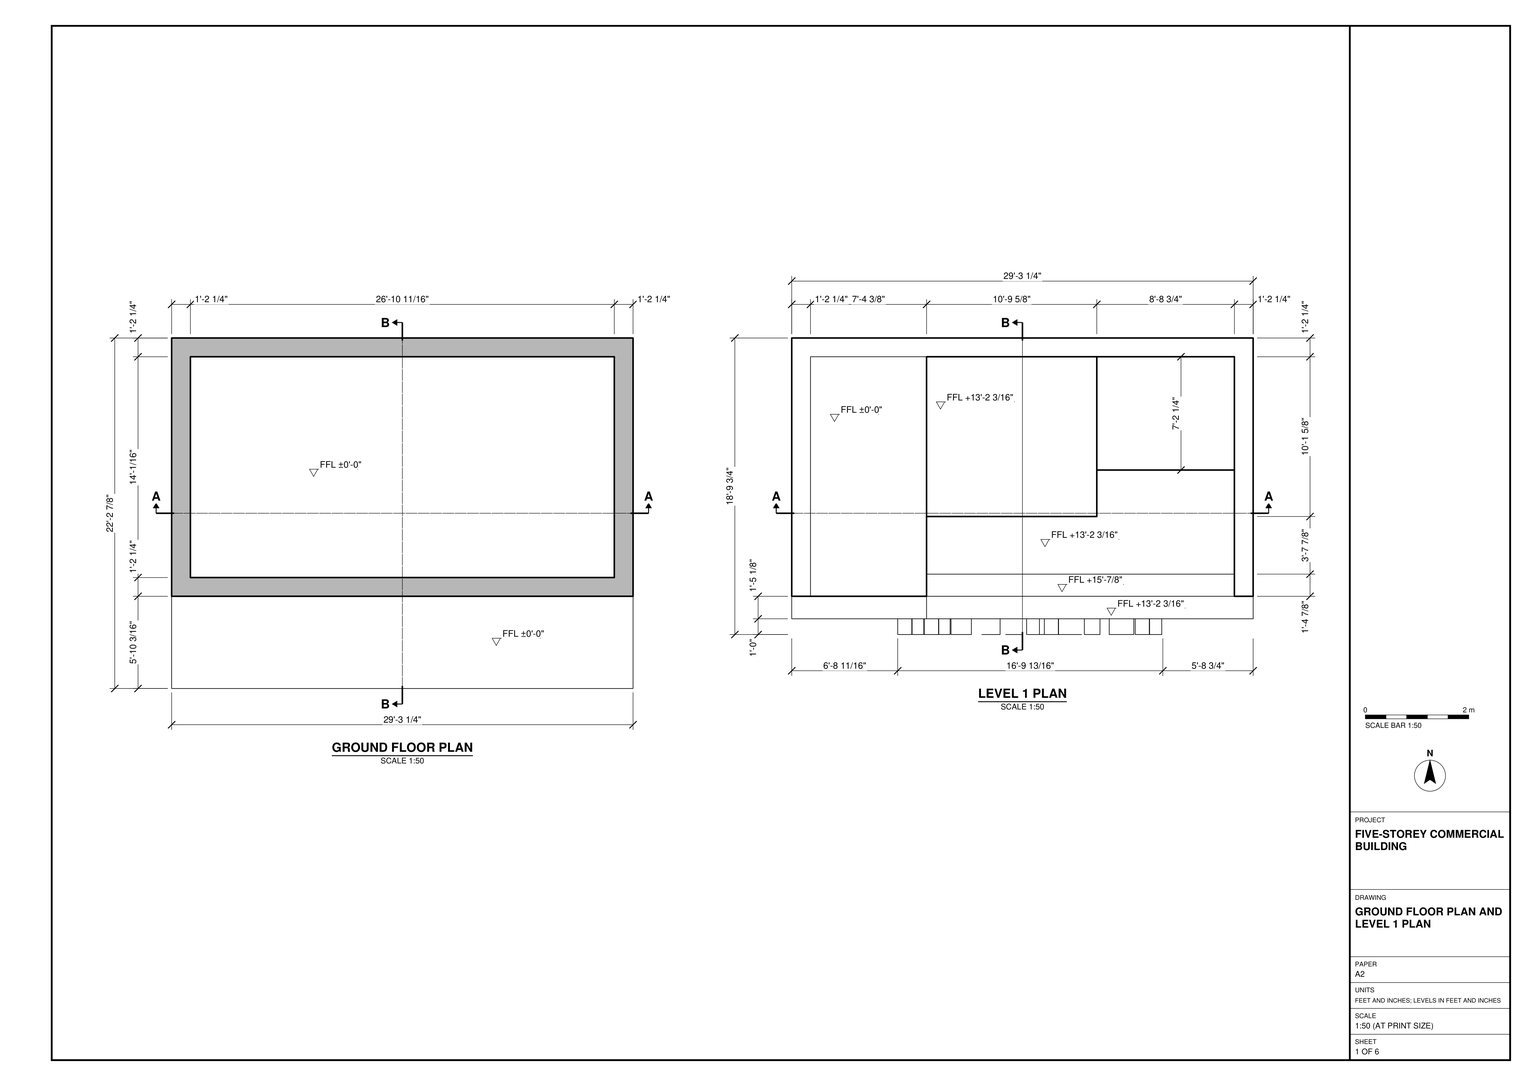
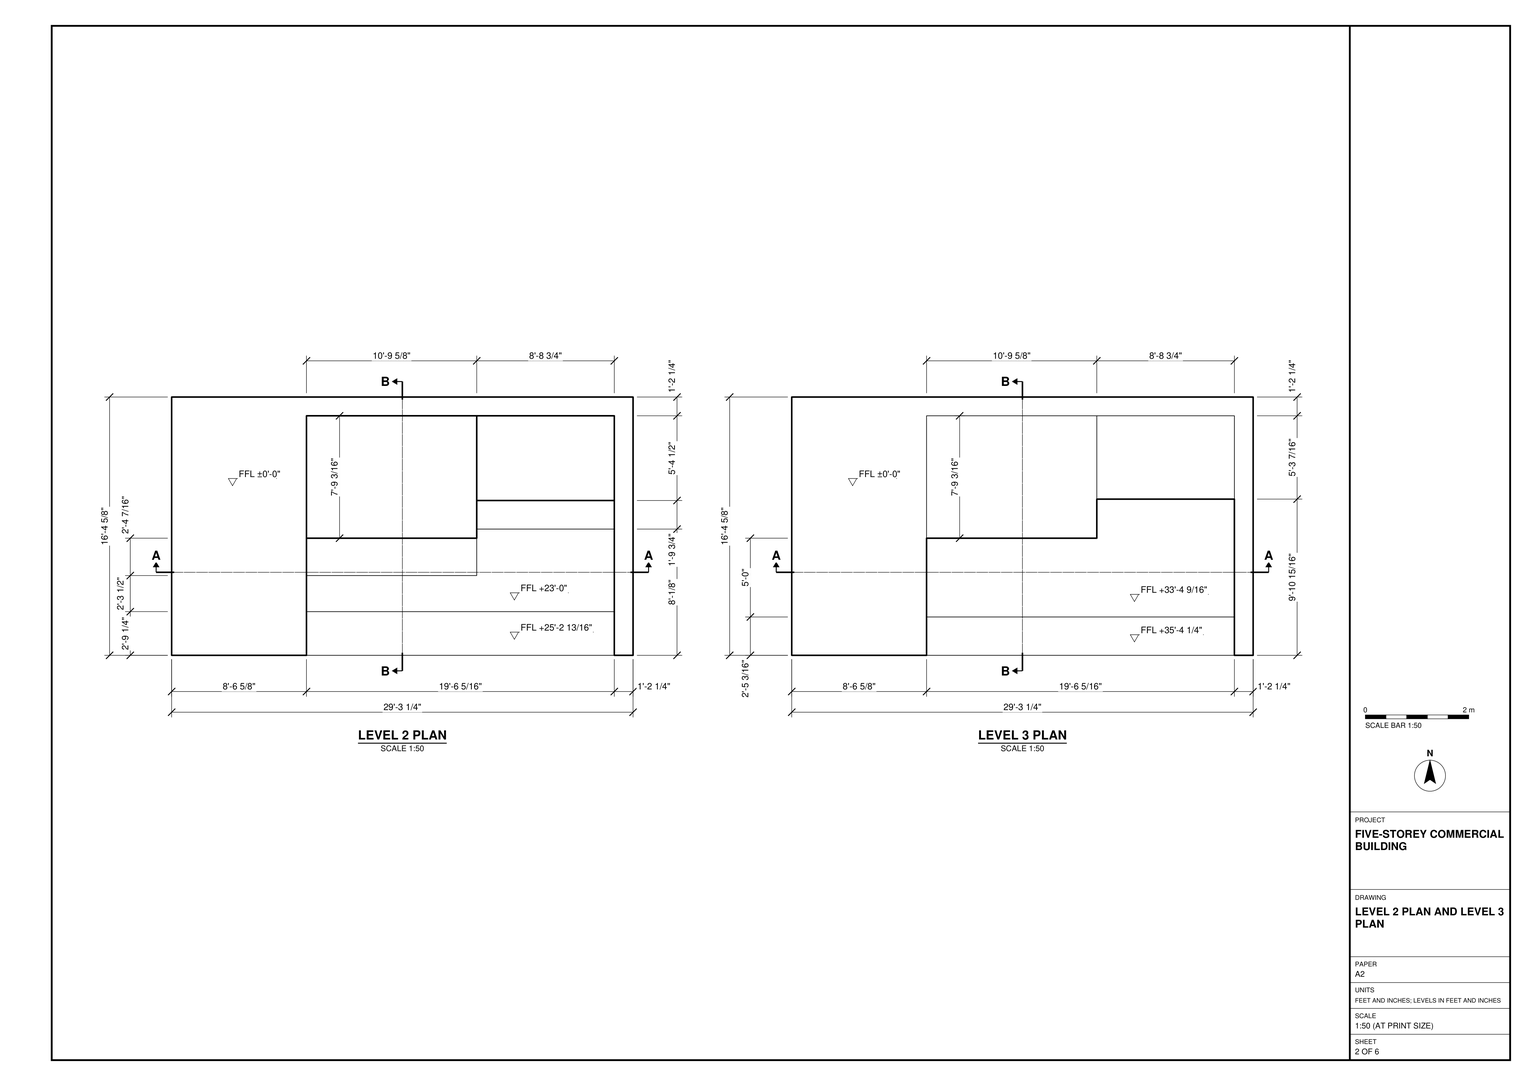
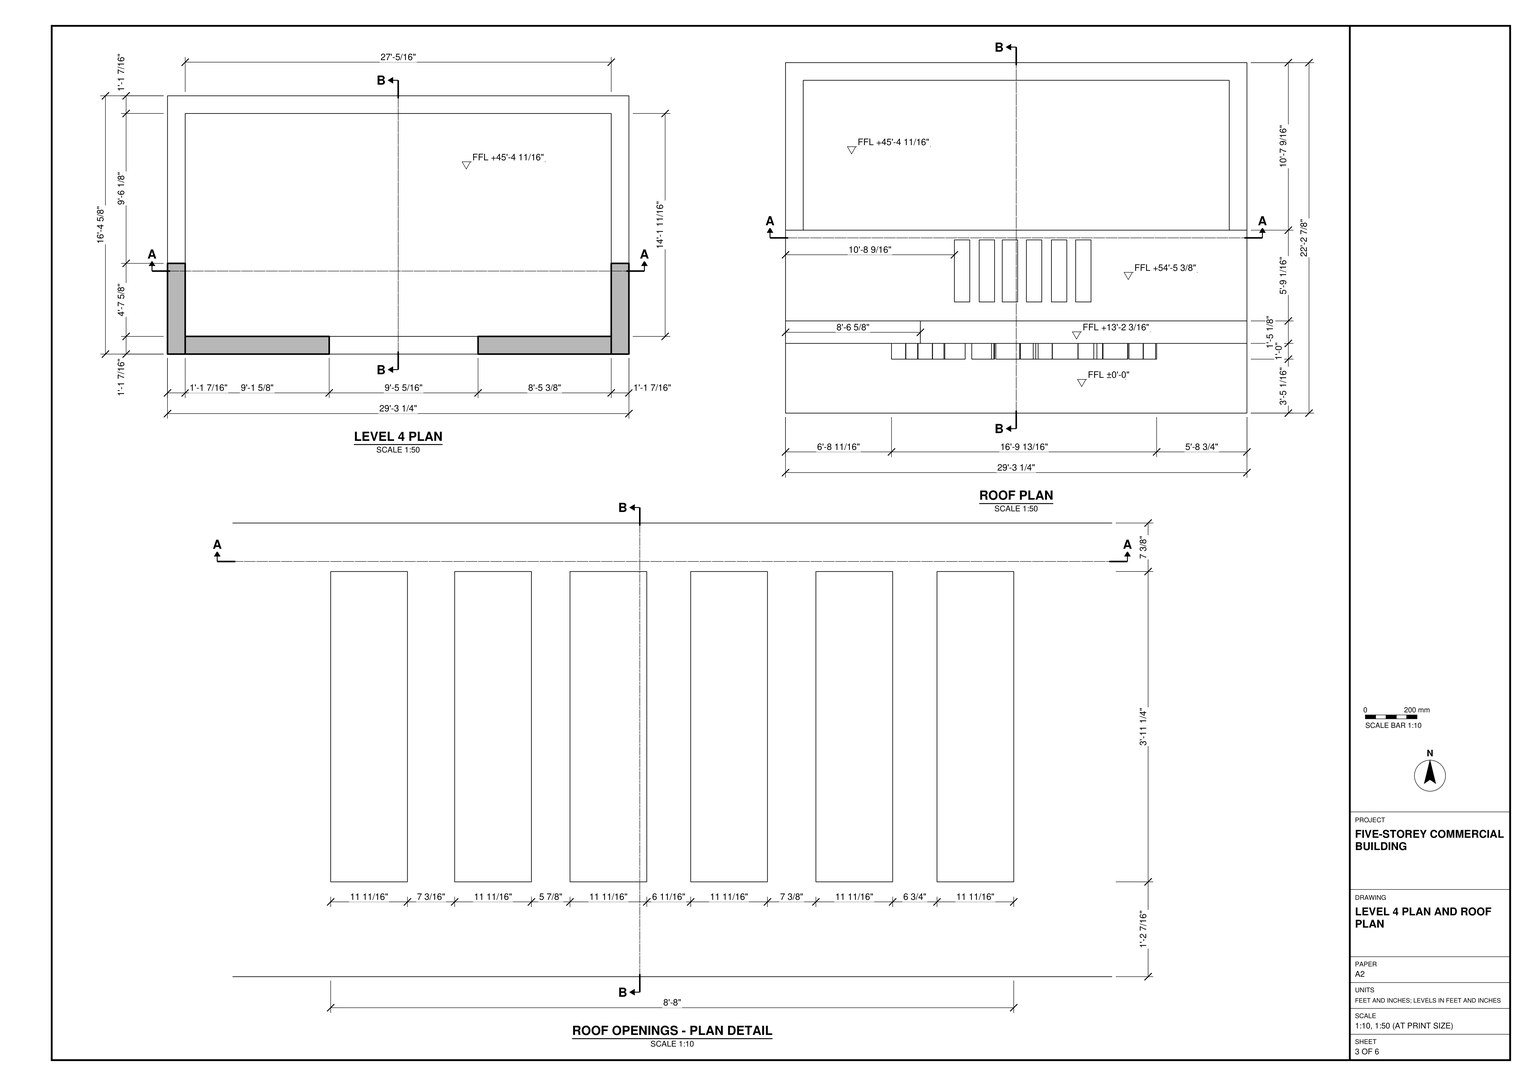
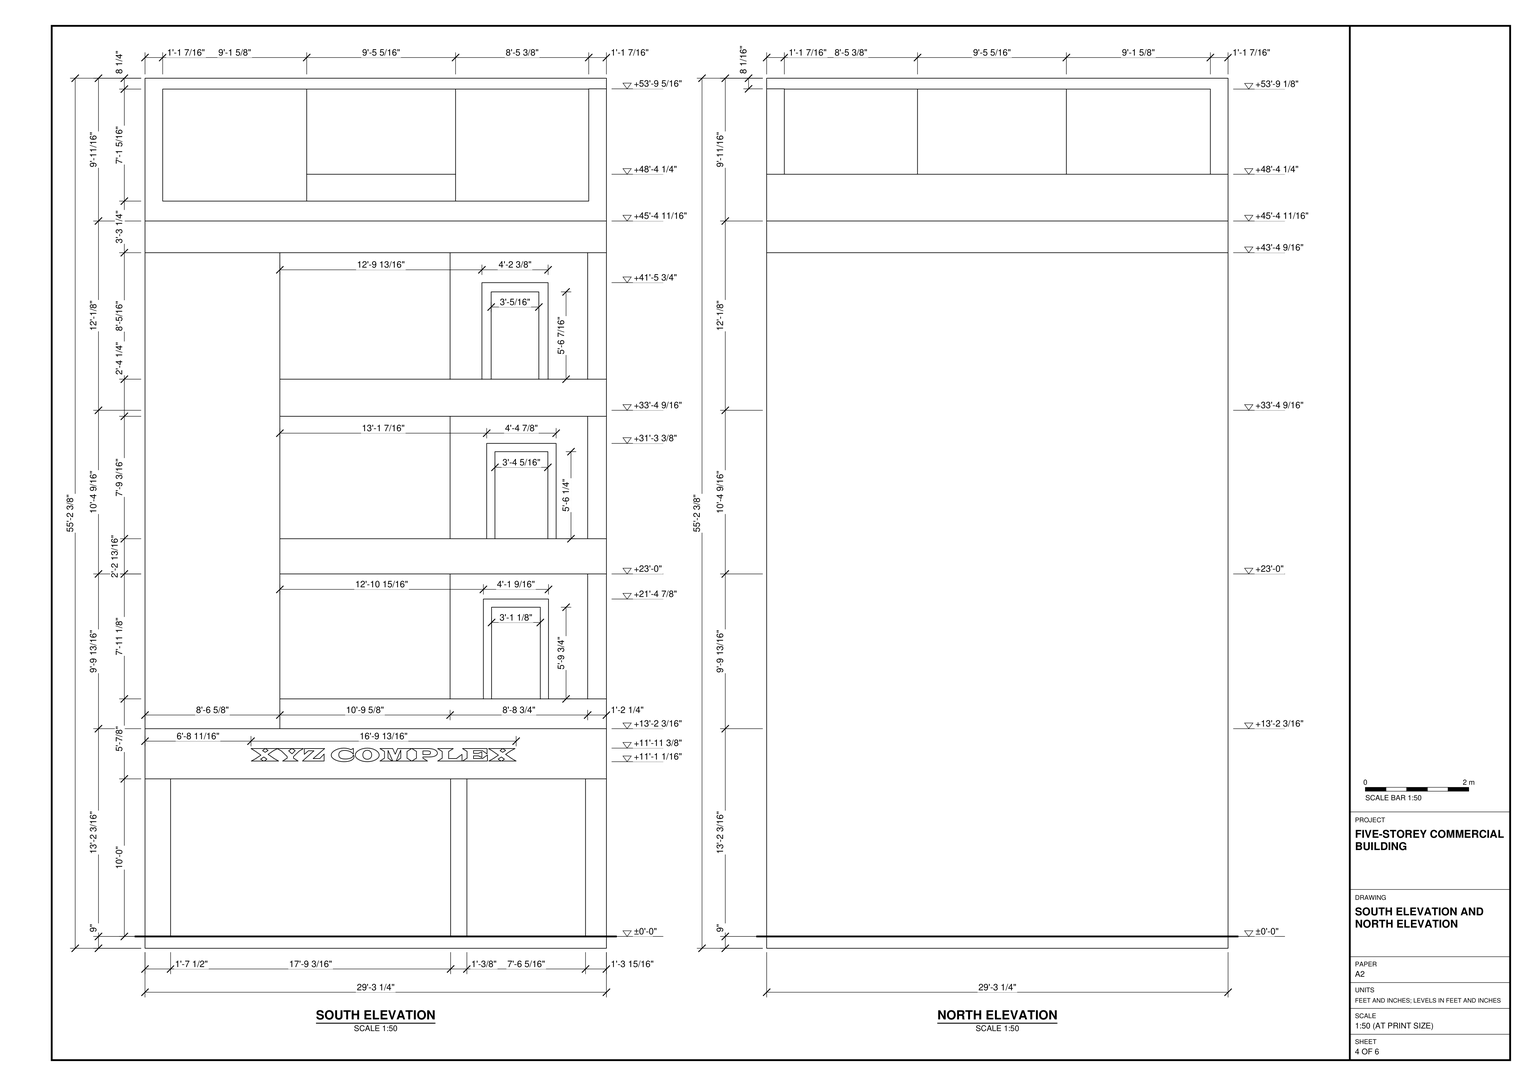
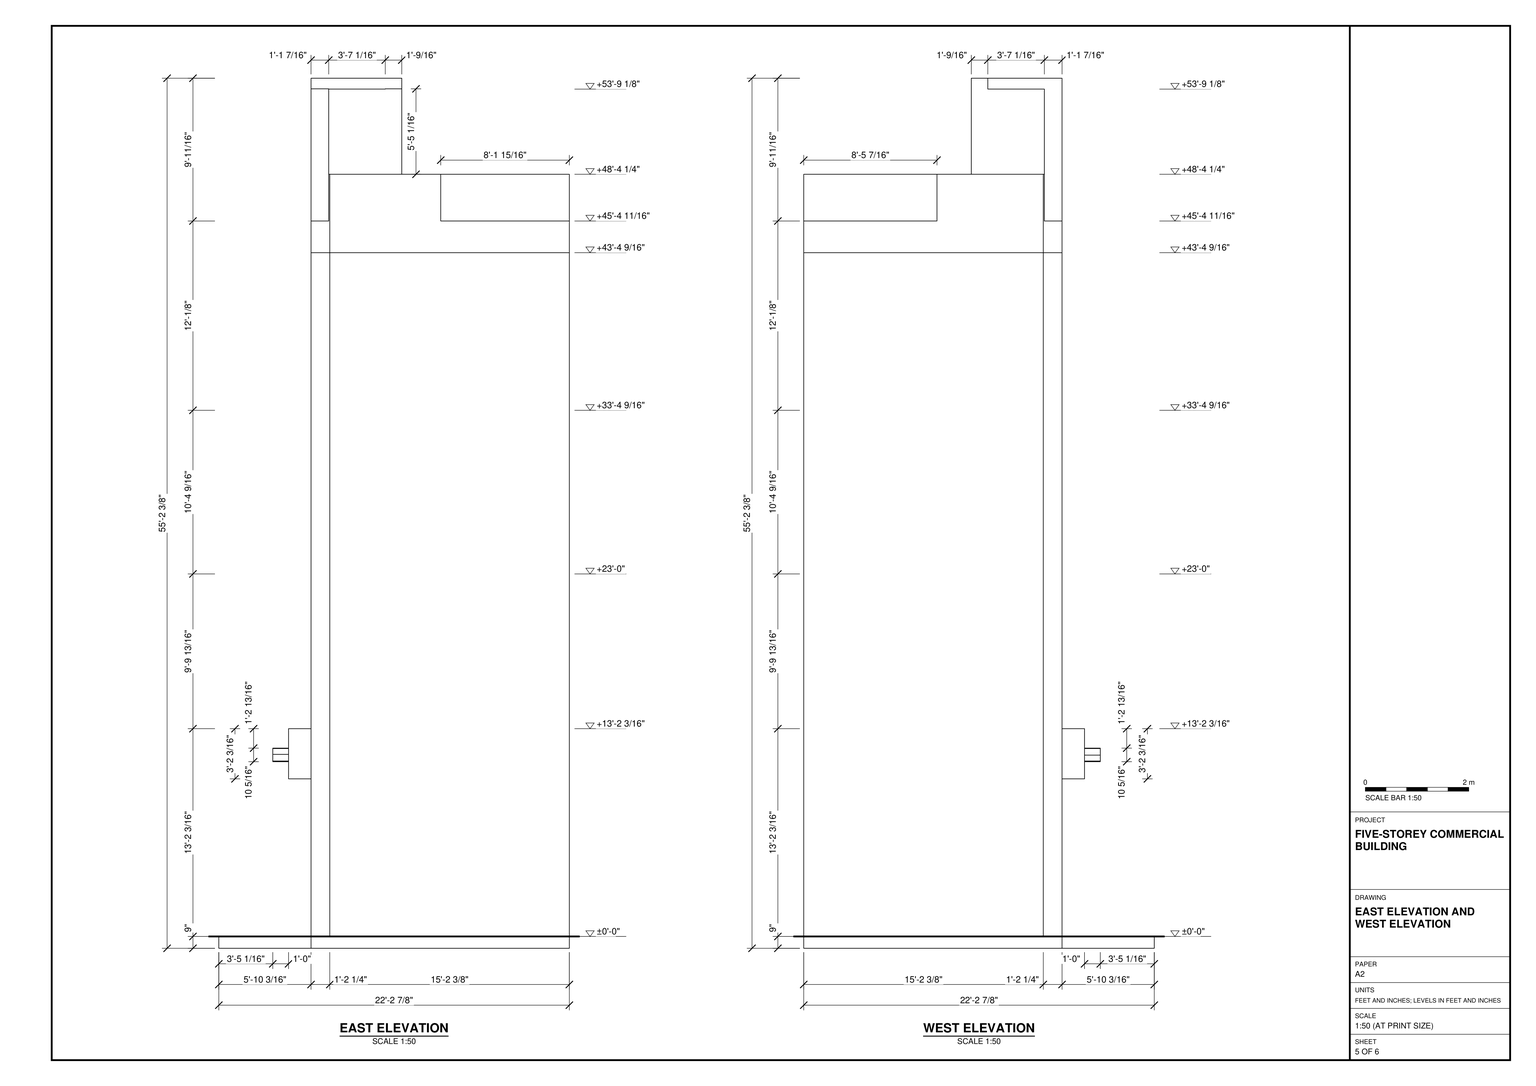
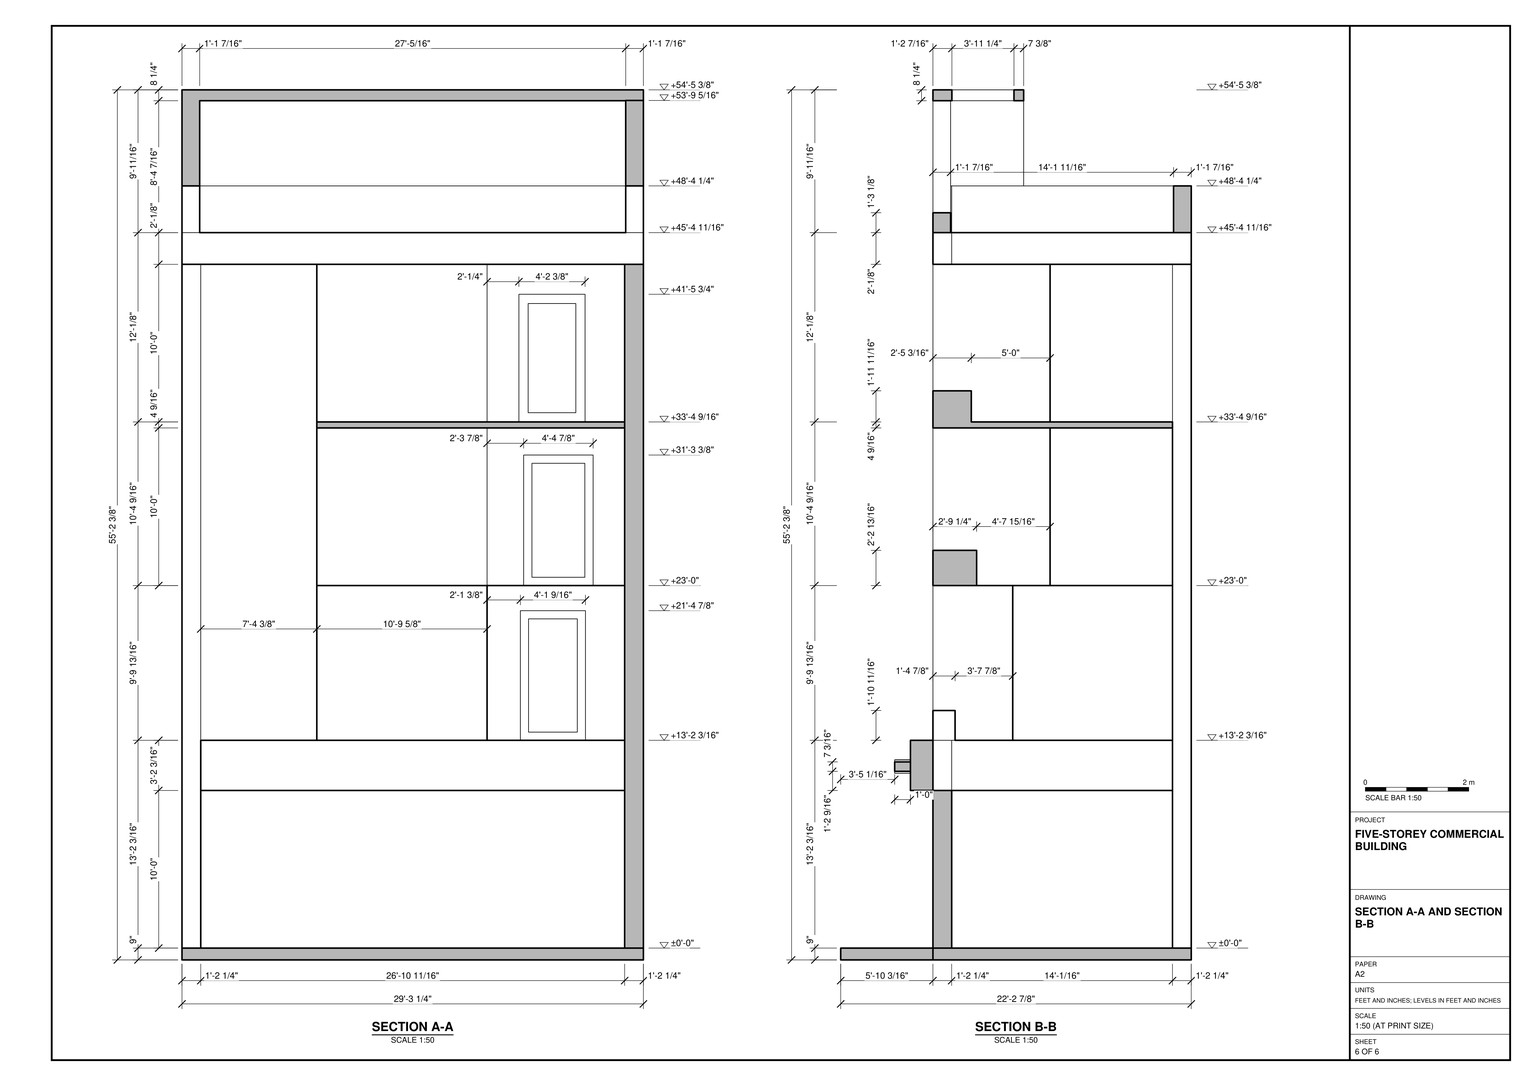
Use task_files/diagram_01.pdf to build the five-storey commercial building in SketchUp. Work in feet and inches. The overall width is 29'-3 1/4" along X, the depth is 22'-2 7/8" along Y, and the height is 55'-2 3/8" along Z. Set the ground floor at ±0'-0" and Levels 1 through 4 at +13'-2 3/16", +23'-0", +33'-4 9/16", and +45'-4 11/16", respectively.

Start with the rectangular ground-floor enclosure and extend the base in front of it as drawn. Use the wall thicknesses shown in plan. Model each slab from its own plan rather than copying a solid floor plate up the building. On Levels 1 through 3, keep the left-hand bay open to the ground floor and follow the changes in depth between the middle and right-hand bays. On Level 4, form the front corner walls and leave the gap between them. Use the enlarged roof detail to cut the six narrow rectangular openings in the front roof strip.

Follow the sheets for openings, stairs, built-in joinery and main furniture wherever shown. Keep walls, slabs, roof elements and each furniture or joinery piece in separate groups or components, and use components for repeated parts. Any decor or loose items shown may be suitable library components. Save one SketchUp model as output_files/five_storey_commercial_building_with_six_roof_openings.skp.

# SketchUp Ruby script. Lengths in inches.
U = 1.inch
M = Sketchup.active_model
def pt(a) = Geom::Point3d.new(a.map { |v| v * U })
def face(e, loops, mat)
  f = e.add_face(loops[0].map { |a| pt(a) })
  loops[1..].each { |l| e.add_face(l.map { |a| pt(a) }).erase! }
  f.material = f.back_material = mat if mat
  f
end
# faces: each face lists its corners as indices into pts; further lists are holes
def faces(e, pts, list, mat = nil) = list.each { |f| face(e, (f[0].is_a?(Array) ? f : [f]).map { |l| l.map { |i| pts[i] } }, mat) }
# xy, xz, yz: faces in a plane at the given z, y or x. An outline is a flat list of corners, or four numbers for a rectangle; further outlines are holes
def ring(l) = l.size == 4 ? [[l[0], l[1]], [l[2], l[1]], [l[2], l[3]], [l[0], l[3]]] : l.each_slice(2).to_a
def flat(e, list, mat, &to3) = list.each { |f| face(e, (f[0].is_a?(Array) ? f : [f]).map { |l| ring(l).map { |u, v| to3.(u, v) } }, mat) }
def xy(e, z, list, mat = nil) = flat(e, list, mat) { |x, y| [x, y, z] }
def xz(e, y, list, mat = nil) = flat(e, list, mat) { |x, z| [x, y, z] }
def yz(e, x, list, mat = nil) = flat(e, list, mat) { |y, z| [x, y, z] }
def lines(e, pts, list) = list.each { |a, b| e.add_line(pt(pts[a]), pt(pts[b])) }
# prism: a flat outline (further loops are holes) pulled along v
def prism(e, loops, v, mat = nil)
  f = face(e, loops, mat); d = Geom::Vector3d.new(v.map { |x| x * U })
  f.pushpull(f.normal.samedirection?(d) ? d.length : -d.length)
end
def box(e, o, s, mat = nil) = prism(e, [[o, [o[0] + s[0], o[1], o[2]], [o[0] + s[0], o[1] + s[1], o[2]], [o[0], o[1] + s[1], o[2]]]], [0, 0, s[2]], mat)
def at(x, y, z, deg = 0) = Geom::Transformation.translation(pt([x, y, z])) * Geom::Transformation.rotation(ORIGIN, Z_AXIS, deg.degrees)
def axes(o, x, y, z) = Geom::Transformation.new([*x, 0, *y, 0, *z, 0, *pt(o).to_a, 1])
def part(name) = M.definitions.add(name)
# library, detail: a bought-in or finely detailed component or shape, given as its bounding box
def library(name, o, s) = part(name).tap { |d| box(d.entities, o, s) }
def detail(e, o, s) = box(e.add_group.entities, o, s)
def put(e, d, t, mat = nil) = e.add_instance(d, t).tap { |i| i.material = mat if mat }
def group(e, t, mat = nil) = e.add_group.tap { |g| g.transformation = t; g.material = mat if mat }.entities
root = M.entities
M.materials.add("[0029_BlanchedAlmond]").color = [255, 235, 205]
M.materials.add("[0035_Tan]").color = [210, 180, 140]
M.materials.add("[0036_BurlyWood]").color = [222, 184, 135]
M.materials.add("[Asphalt New]").color = [67, 60, 62]
M.materials.add("[Basic Tile]").color = [203, 206, 202]
M.materials.add("[Blinds Cellular White]").color = [217, 211, 213]
M.materials.add("[Carpet Diamond Olive]").color = [87, 77, 61]
M.materials.add("[Formica Graystone]").color = [149, 146, 135]
M.materials.add("[Formica Laminate Dark]").color = [50, 53, 60]
M.materials.add("[Formica Laminate Light]").color = [213, 189, 164]
M.materials.add("[Formica Speckled Grey]").color = [94, 105, 111]
M.materials.add("[Leather Blue]").color = [45, 57, 74]
M.materials.add("[Leather Red Brown]").color = [76, 40, 8]
M.materials.add("[Quartz Light Brown]").color = [199, 184, 152]
M.materials.add("[Terrazzo Light Blue]").color = [196, 214, 227]
M.materials.add("[Terrazzo Tile Light]").color = [219, 217, 210]
M.materials.add("[Wood Veneer 01]").color = [81, 47, 25]
M.materials.add("[Wood Veneer 01]1").color = [94, 55, 29]
M.materials.add("[Wood Veneer 01]2").color = [89, 52, 27]
c1 = library("XYZ COMPLEX\#1",[-0.1875,0,0],[201.83,10.32,12])
xy(root,0,[[0,0,351.25,70.21],[0,70.21,351.25,266.85]])
xy(root,9,[[0,70.21,351.25,84.49],[0,84.49,0,266.85,351.25,266.85,351.25,84.49,336.97,84.49,336.97,252.57,14.28,252.57,14.28,84.49],[14.28,84.49,336.97,252.57]])
xy(root,9,[[0,0,351.25,70.21]],"[Terrazzo Light Blue]")
xy(root,129,[[14.28,70.21,336.97,84.49],[14.28,84.49,336.97,252.57]])
xy(root,129,[[0,53.09,19.48,70.21],[19.48,53.09,232.65,70.21],[232.65,53.09,245.03,70.21],[245.03,53.09,335.35,70.21],[335.35,53.09,351.25,70.21]],"[Formica Speckled Grey]")
xy(root,167.1875,[[14.28,70.21,102.64,252.57],[102.64,130.95,232.24,252.57],[232.24,166.32,336.97,252.57]])
xy(root,167.1875,[[0,53.09,102.64,70.21],[102.64,53.09,351.25,70.21]],"[Formica Speckled Grey]")
xy(root,167.1875,[[102.64,87.07,336.97,87.07,336.97,166.32,232.24,166.32,232.24,130.95,102.64,130.95]],"[Leather Blue]")
xy(root,189.875,[[102.64,70.21,336.97,87.07]],"[Formica Laminate Dark]")
xy(root,285,[[102.64,159.38,232.24,252.57],[232.24,188.07,336.97,252.57]])
xy(root,285,[[102.64,70.21,336.97,103.47]],"[Formica Speckled Grey]")
xy(root,285,[[102.64,103.47,336.97,103.47,336.97,166.32,232.24,166.32,232.24,130.95,102.64,130.95],[102.64,130.95,232.24,159.38],[232.24,166.32,336.97,188.07]],"[Leather Red Brown]")
xy(root,311.8125,[[102.64,70.21,336.97,103.47]],"[Formica Speckled Grey]")
xy(root,405,[[102.64,159.38,232.24,252.57],[232.24,188.07,336.97,252.57]])
xy(root,405,[[102.64,70.21,102.64,159.38,232.24,159.38,232.24,188.07,336.97,188.07,336.97,70.21]],"[0029_BlanchedAlmond]")
xy(root,409.5625,[[102.64,159.38,232.24,252.57],[232.24,189.13,336.97,252.57]])
xy(root,409.5625,[[102.64,99.42,336.97,99.42,336.97,189.13,232.24,189.13,232.24,159.38,102.64,159.38]],"[Carpet Diamond Olive]")
xy(root,433.25,[[102.64,70.21,336.97,99.42]],"[Formica Speckled Grey]")
xy(root,529.5625,[[0,70.21,0,266.85,351.25,266.85,351.25,70.21,336.97,70.21,336.97,189.13,232.24,189.13,232.24,159.38,102.64,159.38,102.64,70.21],[232.24,188.07,336.97,189.13]])
xy(root,529.5625,[[102.64,70.21,336.97,159.38],[232.24,159.38,336.97,188.07]],"[0029_BlanchedAlmond]")
xy(root,553.6875,[[0,70.21,351.25,83.68],[0,165.42,0,266.85,351.25,266.85,351.25,168.9375,337.79,168.9375,337.79,253.38,13.47,253.38,13.47,165.42]])
xy(root,553.6875,[[13.47,83.68,337.79,253.38]],"[Terrazzo Tile Light]")
xy(root,568.8125,[[13.47,70.21,123.09,83.68],[236.41,70.21,337.79,83.68]])
xy(root,568.8125,[[123.09,70.21,236.41,83.68]],"[Formica Laminate Dark]")
xy(root,589.25,[[0,83.68,13.47,139.28],[337.79,83.68,351.25,139.28]])
xy(root,589.25,[[0,139.28,13.47,139.28,13.47,253.38,337.79,253.38,337.79,139.28,351.25,139.28,351.25,266.85,0,266.85]],"[Quartz Light Brown]")
xy(root,654.11,[[13.47,70.21,123.09,83.68],[236.41,70.21,337.79,83.68],[337.79,83.68,351.25,126.71]])
xy(root,654.11,[[[123.09,70.21,123.09,83.68,13.47,83.68,13.47,139.28,337.79,139.28,337.79,83.68,236.41,83.68,236.41,70.21],[128.5625,84.65,140.25,131.9],[220.875,84.65,232.5625,131.9],[147.4375,84.65,159.125,131.9],[202.4375,84.65,214.125,131.9],[165,84.65,176.6875,131.9],[183.375,84.65,195.0625,131.9]]],"[Formica Laminate Dark]")
xy(root,654.3125,[[337.79,70.21,351.25,83.68],[337.79,126.71,351.25,139.28]])
xy(root,662.375,[[[0,70.21,351.25,139.28],[128.5625,84.65,140.25,131.9],[147.4375,84.65,159.125,131.9],[165,84.65,176.6875,131.9],[183.375,84.65,195.0625,131.9],[202.4375,84.65,214.125,131.9],[220.875,84.65,232.5625,131.9]]],"[Formica Laminate Dark]")
xz(root,0,[[0,0,351.25,9]],"[Terrazzo Light Blue]")
xz(root,53.09,[[0,129,351.25,167.1875]],"[Formica Speckled Grey]")
xz(root,70.21,[[0,0,351.25,9],[0,129,14.28,167.1875],[14.28,129,336.97,167.1875],[336.97,129,351.25,167.1875]])
xz(root,70.21,[[0,167.1875,102.64,529.5625]],"[Asphalt New]")
xz(root,70.21,[[19.48,9,232.65,129],[245.03,9,335.35,129]],"[Blinds Cellular White]")
xz(root,70.21,[[13.47,568.8125,123.09,654.11],[236.41,568.8125,337.79,654.11]],"[Formica Graystone]")
xz(root,70.21,[[0,9,19.48,129],[232.65,9,245.03,129],[335.35,9,351.25,129],[102.64,167.1875,351.25,189.875],[336.97,189.875,351.25,285],
  [336.97,311.8125,351.25,405],[336.97,433.25,351.25,529.5625],[[0,553.6875,351.25,662.375],[13.47,568.8125,337.79,654.11]]],"[Formica Laminate Dark]")
xz(root,70.21,[[102.64,285,351.25,311.8125],[102.64,405,351.25,433.25],[0,529.5625,351.25,553.6875]],"[Formica Speckled Grey]")
xz(root,83.68,[[0,553.6875,13.47,589.25],[337.79,553.6875,351.25,589.25],[337.79,654.11,351.25,654.3125]])
xz(root,83.68,[[13.47,553.6875,337.79,568.8125],[13.47,568.8125,123.09,589.25],[236.41,568.8125,337.79,589.25],[13.47,589.25,123.09,654.11],[236.41,589.25,337.79,654.11]],"[Formica Graystone]")
xz(root,84.49,[[14.28,9,336.97,129]])
xz(root,84.65,[[128.5625,654.11,140.25,662.375],[147.4375,654.11,159.125,662.375],[165,654.11,176.6875,662.375],[183.375,654.11,195.0625,662.375],[202.4375,654.11,214.125,662.375],
  [220.875,654.11,232.5625,662.375]])
xz(root,87.07,[[102.64,167.1875,336.97,189.875]],"[Formica Speckled Grey]")
xz(root,99.42,[[102.64,409.5625,336.97,433.25]],"[Formica Speckled Grey]")
xz(root,103.47,[[102.64,285,336.97,311.8125]],"[Formica Speckled Grey]")
xz(root,126.71,[[337.79,654.11,351.25,654.3125]])
xz(root,130.95,[[102.64,167.1875,232.24,285]],"[0036_BurlyWood]")
xz(root,131.9,[[128.5625,654.11,140.25,662.375],[147.4375,654.11,159.125,662.375],[165,654.11,176.6875,662.375],[183.375,654.11,195.0625,662.375],[202.4375,654.11,214.125,662.375],
  [220.875,654.11,232.5625,662.375]])
xz(root,139.28,[[0,589.25,0,662.375,351.25,662.375,351.25,654.3125,337.79,654.3125,337.79,654.11,13.47,654.11,13.47,589.25],[337.79,589.25,351.25,654.3125]],"[Formica Laminate Dark]")
xz(root,159.38,[[102.64,285,232.24,405],[102.64,409.5625,232.24,529.5625]],"[0036_BurlyWood]")
xz(root,166.32,[[232.24,167.1875,257.59,167.1875,257.59,265.875,307.15,265.875,307.15,167.1875,336.97,167.1875,336.97,285,232.24,285]],"[0035_Tan]")
xz(root,166.32,[[263.82,173.42,300.92,259.64]],"[Formica Laminate Light]")
xz(root,166.32,[[[257.59,167.1875,307.15,265.875],[263.82,173.42,300.92,259.64]]],"[Wood Veneer 01]2")
xz(root,188.07,[[232.24,285,260.09,285,260.09,384.375,312.97,384.375,312.97,285,336.97,285,336.97,405,232.24,405]],"[0035_Tan]")
xz(root,188.07,[[266.39,291.3,306.67,378.08]],"[Formica Laminate Light]")
xz(root,188.07,[[[260.09,285,312.97,384.375],[266.39,291.3,306.67,378.08]]],"[Wood Veneer 01]1")
xz(root,189.13,[[232.24,409.5625,256.47,409.5625,256.47,506.75,306.85,506.75,306.85,409.5625,336.97,409.5625,336.97,529.5625,232.24,529.5625]],"[0035_Tan]")
xz(root,189.13,[[263.51,416.6,299.8125,499.72]],"[Formica Laminate Light]")
xz(root,189.13,[[[256.47,409.5625,306.85,506.75],[263.51,416.6,299.8125,499.72]]],"[Wood Veneer 01]")
xz(root,252.57,[[14.28,9,336.97,129],[14.28,129,336.97,167.1875],[102.64,167.1875,232.24,285],[232.24,167.1875,336.97,285],[102.64,285,232.24,405],
  [232.24,285,336.97,405],[102.64,405,232.24,409.5625],[232.24,405,336.97,409.5625]])
xz(root,253.38,[[13.47,553.6875,337.79,589.25]],"[Formica Graystone]")
xz(root,266.85,[[0,0,351.25,9]])
xz(root,266.85,[[0,9,351.25,529.5625]],"[Basic Tile]")
xz(root,266.85,[[0,529.5625,351.25,553.6875],[0,553.6875,351.25,589.25]],"[Quartz Light Brown]")
yz(root,0,[[84.49,9,266.85,529.5625]],"[Basic Tile]")
yz(root,0,[[70.21,9,84.49,529.5625]],"[Formica Laminate Dark]")
yz(root,0,[[53.09,129,70.21,167.1875]],"[Formica Speckled Grey]")
yz(root,0,[[70.21,529.5625,70.21,553.6875,83.68,553.6875,83.68,589.25,84.49,589.25,84.49,529.5625],[84.49,529.5625,84.49,589.25,165.42,589.25,165.42,553.6875,266.85,553.6875,266.85,529.5625],[70.21,553.6875,70.21,662.375,126.71,662.375,126.71,654.11,83.68,654.11,83.68,553.6875],[165.42,553.6875,266.85,589.25],[83.68,589.25,83.68,654.11,126.71,654.11,126.71,662.375,139.28,662.375,139.28,589.25]],"[Quartz Light Brown]")
yz(root,0,[[0,0,70.21,9],[70.21,0,266.85,9]],"[Terrazzo Light Blue]")
yz(root,13.47,[[83.68,553.6875,84.49,589.25],[70.21,568.8125,83.68,654.11]])
yz(root,13.47,[[84.49,553.6875,253.38,589.25],[83.68,589.25,139.28,654.11]],"[Formica Graystone]")
yz(root,14.28,[[84.49,9,252.57,129],[70.21,129,84.49,167.1875],[84.49,129,252.57,167.1875]])
yz(root,102.64,[[70.21,167.1875,87.07,189.875],[130.95,167.1875,252.57,285],[70.21,285,103.47,311.8125],[159.38,285,252.57,405],[70.21,405,70.21,433.25,99.42,433.25,99.42,409.5625,159.38,409.5625,159.38,405],
  [159.38,405,252.57,409.5625]])
yz(root,102.64,[[87.07,167.1875,130.95,167.1875,130.95,285,70.21,285,70.21,189.875,87.07,189.875],[103.47,285,159.38,285,159.38,405,70.21,405,70.21,311.8125,103.47,311.8125],[99.42,409.5625,159.38,409.5625,159.38,529.5625,70.21,529.5625,70.21,433.25,99.42,433.25]],"[0036_BurlyWood]")
yz(root,123.09,[[70.21,568.8125,83.68,654.11]],"[Formica Graystone]")
yz(root,128.5625,[[84.65,654.11,131.9,662.375]])
yz(root,140.25,[[84.65,654.11,131.9,662.375]])
yz(root,147.4375,[[84.65,654.11,131.9,662.375]])
yz(root,159.125,[[84.65,654.11,131.9,662.375]])
yz(root,165,[[84.65,654.11,131.9,662.375]])
yz(root,176.6875,[[84.65,654.11,131.9,662.375]])
yz(root,183.375,[[84.65,654.11,131.9,662.375]])
yz(root,195.0625,[[84.65,654.11,131.9,662.375]])
yz(root,202.4375,[[84.65,654.11,131.9,662.375]])
yz(root,214.125,[[84.65,654.11,131.9,662.375]])
yz(root,220.875,[[84.65,654.11,131.9,662.375]])
yz(root,232.24,[[166.32,167.1875,252.57,285],[188.07,285,252.57,405]])
yz(root,232.24,[[130.95,167.1875,166.32,285],[159.38,285,188.07,405],[159.38,409.5625,189.13,529.5625]],"[0036_BurlyWood]")
yz(root,232.5625,[[84.65,654.11,131.9,662.375]])
yz(root,236.41,[[70.21,568.8125,83.68,654.11]],"[Formica Graystone]")
yz(root,336.97,[[84.49,9,252.57,129],[84.49,129,252.57,129,252.57,167.1875,87.07,167.1875,87.07,189.875,84.49,189.875],[166.32,167.1875,252.57,285],[188.07,285,252.57,405],[84.49,405,87.07,433.25],
  [87.07,405,159.38,405,159.38,409.5625,99.42,409.5625,99.42,433.25,87.07,433.25],[159.38,405,166.32,409.5625],[166.32,405,188.07,409.5625],[188.07,405,252.57,409.5625],[188.07,409.5625,189.13,529.5625]])
yz(root,336.97,[[87.07,167.1875,87.07,189.875,84.49,189.875,84.49,285,166.32,285,166.32,167.1875],[70.21,189.875,84.49,285],[103.47,285,103.47,311.8125,70.21,311.8125,70.21,405,166.32,405,166.32,285],[166.32,285,188.07,405],[99.42,409.5625,99.42,433.25,70.21,433.25,70.21,529.5625,188.07,529.5625,188.07,409.5625]],"[0029_BlanchedAlmond]")
yz(root,337.79,[[83.68,553.6875,84.49,589.25],[70.21,568.8125,83.68,654.11],[70.21,654.11,83.68,654.3125],[126.71,654.11,139.28,654.3125]])
yz(root,337.79,[[84.49,553.6875,253.38,589.25],[83.68,589.25,139.28,654.11]],"[Formica Graystone]")
yz(root,351.25,[[84.49,9,266.85,529.5625]],"[Basic Tile]")
yz(root,351.25,[[70.21,9,84.49,529.5625],[53.09,129,70.21,167.1875],[70.21,529.5625,84.49,529.5625,84.49,589.25,83.68,589.25,83.68,553.6875,70.21,553.6875]],"[Formica Speckled Grey]")
yz(root,351.25,[[84.49,529.5625,266.85,529.5625,266.85,553.6875,168.9375,553.6875,168.9375,589.25,84.49,589.25],[70.21,553.6875,83.68,654.3125],[168.9375,553.6875,266.85,589.25],[83.68,589.25,139.28,589.25,139.28,654.3125,126.71,654.3125,126.71,654.11,83.68,654.11],[83.68,654.11,126.71,654.11,126.71,654.3125,139.28,654.3125,139.28,662.375,70.21,662.375,70.21,654.3125,83.68,654.3125]],"[Quartz Light Brown]")
yz(root,351.25,[[0,0,70.21,9],[70.21,0,266.85,9]],"[Terrazzo Light Blue]")
p = [[14.28,252.57,167.1875],[14.28,252.57,529.5625],[14.28,84.49,167.1875],[14.28,84.49,529.5625]]
lines(root,p,[[0,1],[2,3]])
put(root,c1,axes([80.87,53.09,142.06],[1,0,0],[0,0,1],[0,-1,0]))
